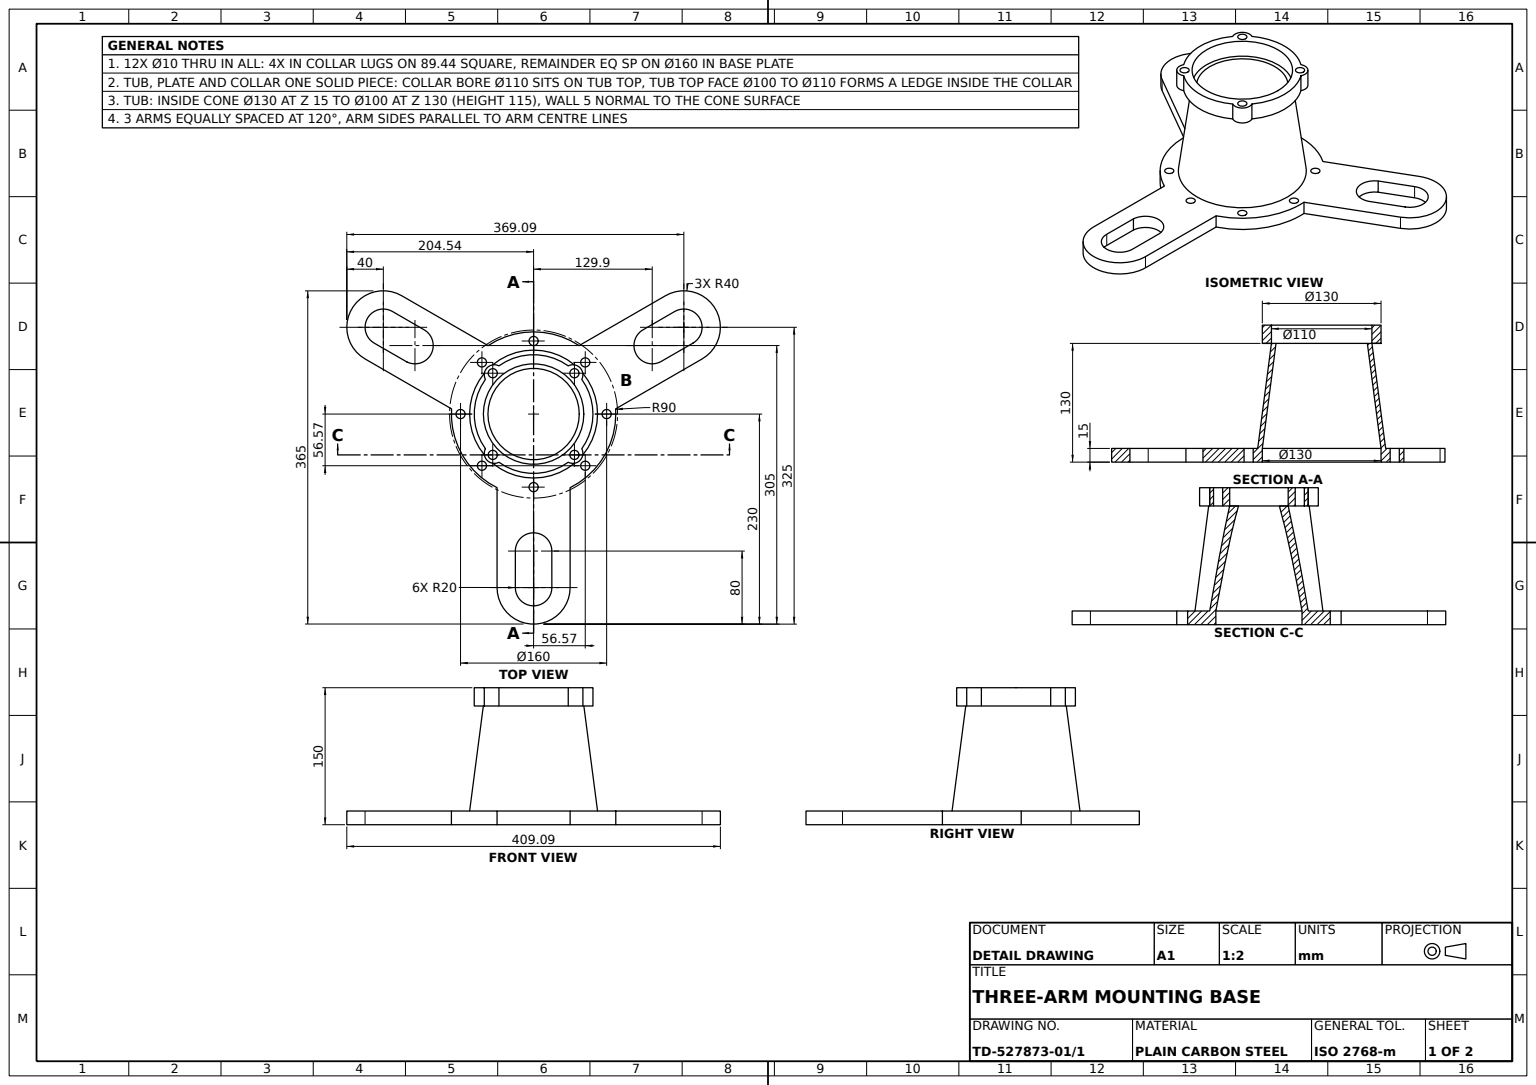
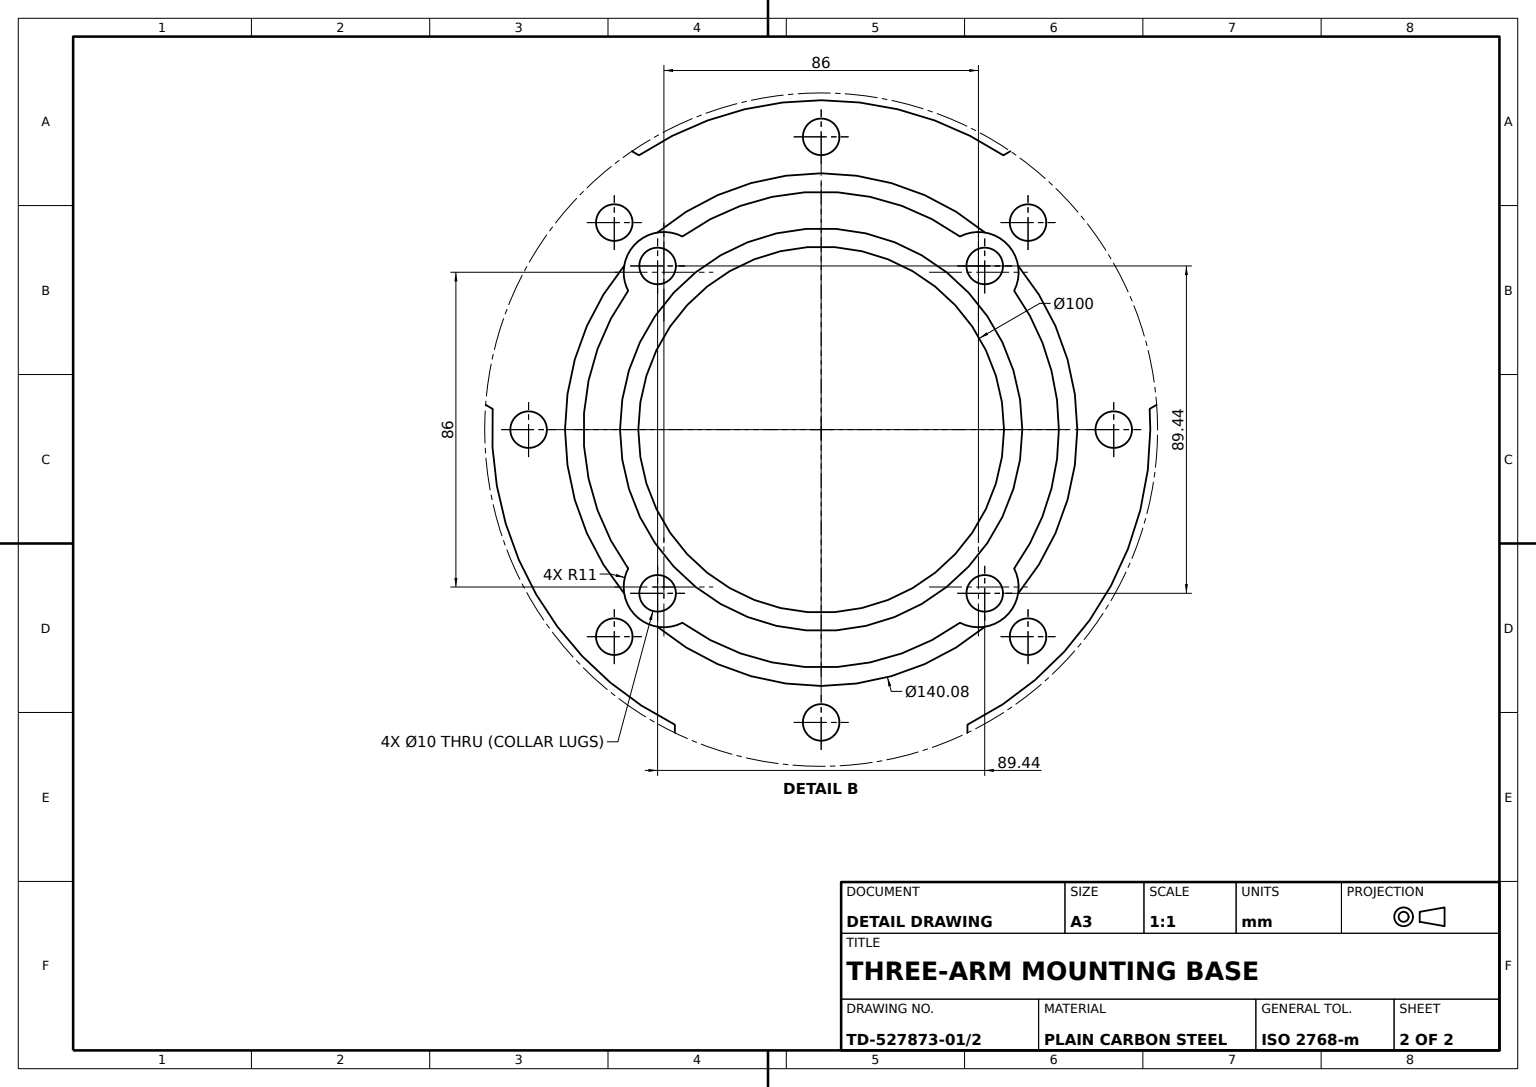
solid
v1 (-129.641016,15,-144.544827)
v2 (-74.952305,15,-49.8212)
e1 v1 v2 LINE
v3 (-129.641016,0,-144.544827)
e2 v1 v3 LINE
v4 (-74.952305,0,-49.8212)
e3 v3 v4 LINE
e4 v2 v4 LINE
face PLANE(AX(P(-34.641016,15,20),D(0.866025404,0,-0.5),D(-0.5,0,-0.866025404))) rev [-e1 e2 e3 -e4]
v5 (43,130,54)
v6 (43,150,54)
e5 v5 v6 LINE
v7 (52.771822,130,37.949109)
e6 v5 v7 CIRCLE(AX(P(43,130,43),D(0,1,0),D(-1,0,0)),11)
v8 (52.771822,150,37.949109)
e7 v8 v7 LINE
e8 v6 v8 CIRCLE(AX(P(43,150,43),D(0,1,0),D(-1,0,0)),11)
face CYL(AX(P(43,130,43),D(0,1,0),D(0,0,1)),11) [-e5 e6 -e7 -e8]
v9 (56.568542,0,-51.568542)
v10 (56.568542,15,-51.568542)
e9 v9 v10 LINE
v11 (56.568542,0,-61.568542)
e10 v11 v9 CIRCLE(AX(P(56.568542,0,-56.568542),D(0,1,0),D(0,0,1)),5)
v12 (56.568542,15,-61.568542)
e11 v11 v12 LINE
e12 v12 v10 CIRCLE(AX(P(56.568542,15,-56.568542),D(0,1,0),D(0,0,1)),5)
face CYL(AX(P(56.568542,-47,-56.568542),D(0,1,0),D(0,0,1)),5) rev [-e9 -e10 e11 e12]
v13 (0,130,-50)
v14 (0,130,50)
e13 v13 v14 CIRCLE(AX(P(0,130,0),D(0,1,0),D(0,0,1)),50)
e14 v14 v13 CIRCLE(AX(P(0,130,0),D(0,1,0),D(0,0,1)),50)
v15 (0,130,55)
v16 (0,130,-55)
e15 v15 v16 CIRCLE(AX(P(0,130,0),D(0,-1,0),D(0,0,1)),55)
e16 v16 v15 CIRCLE(AX(P(0,130,0),D(0,-1,0),D(0,0,1)),55)
face PLANE(AX(P(0,130,0),D(0,1,0),D(0,0,1))) [-e13 -e14] [-e15 -e16]
v17 (0,150,-55)
e17 v17 v16 LINE
v18 (0,150,55)
e18 v17 v18 CIRCLE(AX(P(0,150,0),D(0,1,0),D(1,0,0)),55)
e19 v18 v15 LINE
face CYL(AX(P(0,150,0),D(0,-1,0),D(0,0,-1)),55) rev [-e17 e18 e19 e15]
v19 (-44.722153,130,-49.722153)
v20 (-44.722153,150,-49.722153)
e20 v19 v20 LINE
v21 (-44.722153,130,-39.722153)
e21 v21 v19 CIRCLE(AX(P(-44.722153,130,-44.722153),D(0,1,0),D(0,0,1)),5)
v22 (-44.722153,150,-39.722153)
e22 v21 v22 LINE
e23 v22 v20 CIRCLE(AX(P(-44.722153,150,-44.722153),D(0,1,0),D(0,0,1)),5)
face CYL(AX(P(-44.722153,115,-44.722153),D(0,1,0),D(0,0,1)),5) rev [-e20 -e21 e22 e23]
v23 (148.666667,15,-19.955506)
v24 (148.666667,0,-19.955506)
e24 v23 v24 LINE
v25 (189.956941,0,-19.999954)
e25 v24 v25 LINE
v26 (189.956941,15,-19.999954)
e26 v26 v25 LINE
e27 v23 v26 LINE
face PLANE(AX(P(-0.021309,15,-19.795448),D(-0.001076466,0,-0.999999421),D(-0.999999421,0,0.001076466))) rev [e24 e25 -e26 -e27]
v27 (190,0,-20)
e28 v27 v25 CIRCLE(AX(P(190,0,0),D(0,1,0),D(0,0,1)),20)
v28 (190,15,-20)
e29 v28 v27 LINE
e30 v28 v26 CIRCLE(AX(P(190,15,0),D(0,1,0),D(0,0,1)),20)
face CYL(AX(P(190,15,0),D(0,-1,0),D(0,0,-1)),20) rev [-e28 -e29 e30 e26]
v29 (190,15,-40)
v30 (190,0,-40)
e31 v29 v30 LINE
v31 (190,15,40)
e32 v31 v29 CIRCLE(AX(P(190,15,0),D(0,1,0),D(0,0,1)),40)
v32 (190,0,40)
e33 v31 v32 LINE
e34 v32 v30 CIRCLE(AX(P(190,0,0),D(0,1,0),D(0,0,1)),40)
face CYL(AX(P(190,15,0),D(0,-1,0),D(0,0,-1)),40) [-e31 -e32 e33 e34]
v33 (-57.051358,15,-138.726863)
v34 (-57.051358,0,-138.726863)
e35 v33 v34 LINE
v35 (-91.615309,0,-118.771357)
e36 v35 v34 CIRCLE(AX(P(-75,0,-129.903811),D(0,1,0),D(0,0,1)),20)
v36 (-91.615309,15,-118.771357)
e37 v36 v35 LINE
e38 v36 v33 CIRCLE(AX(P(-75,15,-129.903811),D(0,1,0),D(0,0,1)),20)
face CYL(AX(P(-75,15,-129.903811),D(0,-1,0),D(0,0,-1)),20) rev [e35 -e36 -e37 e38]
v37 (0,0,-65)
v38 (0,0,65)
e39 v37 v38 CIRCLE(AX(P(0,0,0),D(0,1,0),D(0,0,1)),65)
v39 (0,15,-65)
e40 v37 v39 LINE
v40 (0,15,65)
e41 v39 v40 CIRCLE(AX(P(0,15,0),D(0,1,0),D(0,0,1)),65)
e42 v38 v40 LINE
face CYL(AX(P(0,-5,0),D(0,1,0),D(0,0,1)),65) rev [-e39 e40 e41 -e42]
v41 (-112.298939,15,154.50756)
v42 (-112.298939,0,154.50756)
e43 v41 v42 LINE
v43 (-77.658003,15,174.507514)
e44 v41 v43 CIRCLE(AX(P(-95,15,164.544827),D(0,1,0),D(0,0,1)),20)
v44 (-77.658003,0,174.507514)
e45 v43 v44 LINE
e46 v42 v44 CIRCLE(AX(P(-95,0,164.544827),D(0,1,0),D(0,0,1)),20)
face CYL(AX(P(-95,15,164.544827),D(0,-1,0),D(0,0,-1)),20) rev [-e43 e44 e45 -e46]
v45 (52.771822,130,-37.949109)
v46 (52.771822,150,-37.949109)
e47 v45 v46 LINE
e48 v8 v46 CIRCLE(AX(P(0,150,0),D(0,1,0),D(0,0,1)),65)
e49 v7 v45 CIRCLE(AX(P(0,130,0),D(0,1,0),D(0,0,1)),65)
face CYL(AX(P(0,150,0),D(0,-1,0),D(0,0,-1)),65) [e47 -e48 e7 e49]
v47 (-77.658003,0,-174.507514)
e50 v34 v47 LINE
v48 (-77.658003,15,-174.507514)
e51 v33 v48 LINE
e52 v48 v47 LINE
face PLANE(AX(P(17.154016,15,-9.87927),D(-0.866563135,0,0.499067464),D(0.499067464,0,0.866563135))) [-e50 -e35 e51 e52]
v49 (-56.568542,0,51.568542)
v50 (-56.568542,15,51.568542)
e53 v49 v50 LINE
v51 (-56.568542,0,61.568542)
e54 v51 v49 CIRCLE(AX(P(-56.568542,0,56.568542),D(0,1,0),D(0,0,1)),5)
v52 (-56.568542,15,61.568542)
e55 v51 v52 LINE
e56 v52 v50 CIRCLE(AX(P(-56.568542,15,56.568542),D(0,1,0),D(0,0,1)),5)
face CYL(AX(P(-56.568542,-47,56.568542),D(0,1,0),D(0,0,1)),5) rev [-e53 -e54 e55 e56]
v53 (37.949109,150,-52.771822)
v54 (37.949109,130,-52.771822)
e57 v53 v54 LINE
e58 v46 v53 CIRCLE(AX(P(43,150,-43),D(0,1,0),D(0,0,1)),11)
e59 v45 v54 CIRCLE(AX(P(43,130,-43),D(0,1,0),D(0,0,1)),11)
face CYL(AX(P(43,130,-43),D(0,1,0),D(0,0,1)),11) [-e57 -e58 -e47 e59]
v55 (-112.298939,15,-154.50756)
v56 (-112.298939,0,-154.50756)
e60 v55 v56 LINE
e61 v36 v55 LINE
e62 v35 v56 LINE
face PLANE(AX(P(-17.132707,15,9.916178),D(-0.865486669,0,0.500931957),D(0.500931957,0,0.865486669))) rev [-e60 -e61 e37 e62]
v57 (37.949109,130,52.771822)
v58 (37.949109,150,52.771822)
e63 v57 v58 LINE
e64 v57 v5 CIRCLE(AX(P(43,130,43),D(0,1,0),D(-1,0,0)),11)
e65 v58 v6 CIRCLE(AX(P(43,150,43),D(0,1,0),D(-1,0,0)),11)
face CYL(AX(P(43,130,43),D(0,1,0),D(0,0,1)),11) [-e63 e64 e5 -e65]
v59 (56.568542,0,51.568542)
v60 (56.568542,0,61.568542)
e66 v59 v60 CIRCLE(AX(P(56.568542,0,56.568542),D(0,1,0),D(0,0,1)),5)
v61 (56.568542,15,51.568542)
e67 v59 v61 LINE
v62 (56.568542,15,61.568542)
e68 v61 v62 CIRCLE(AX(P(56.568542,15,56.568542),D(0,1,0),D(0,0,1)),5)
e69 v60 v62 LINE
face CYL(AX(P(56.568542,-47,56.568542),D(0,1,0),D(0,0,1)),5) rev [-e66 e67 e68 -e69]
v63 (0,0,-75)
v64 (0,15,-75)
e70 v63 v64 LINE
v65 (0,15,-85)
e71 v64 v65 CIRCLE(AX(P(0,15,-80),D(0,1,0),D(0,0,1)),5)
v66 (0,0,-85)
e72 v66 v65 LINE
e73 v63 v66 CIRCLE(AX(P(0,0,-80),D(0,1,0),D(0,0,1)),5)
face CYL(AX(P(0,-47,-80),D(0,1,0),D(0,0,1)),5) rev [e70 e71 -e72 -e73]
v67 (44.722153,130,-49.722153)
v68 (44.722153,130,-39.722153)
e74 v67 v68 CIRCLE(AX(P(44.722153,130,-44.722153),D(0,1,0),D(0,0,1)),5)
v69 (44.722153,150,-49.722153)
e75 v67 v69 LINE
v70 (44.722153,150,-39.722153)
e76 v69 v70 CIRCLE(AX(P(44.722153,150,-44.722153),D(0,1,0),D(0,0,1)),5)
e77 v68 v70 LINE
face CYL(AX(P(44.722153,115,-44.722153),D(0,1,0),D(0,0,1)),5) rev [-e74 e75 e76 -e77]
v71 (0,130,55.042354)
v72 (0,130,-55.042354)
e78 v71 v72 CIRCLE(AX(P(0,130,0),D(0,1,0),D(0,0,1)),55.042354)
e79 v72 v71 CIRCLE(AX(P(0,130,0),D(0,1,0),D(0,0,1)),55.042354)
e80 v68 v67 CIRCLE(AX(P(44.722153,130,-44.722153),D(0,1,0),D(0,0,1)),5)
v73 (44.722153,130,49.722153)
v74 (44.722153,130,39.722153)
e81 v73 v74 CIRCLE(AX(P(44.722153,130,44.722153),D(0,1,0),D(0,0,1)),5)
e82 v74 v73 CIRCLE(AX(P(44.722153,130,44.722153),D(0,1,0),D(0,0,1)),5)
v75 (-37.949109,130,52.771822)
e83 v75 v57 CIRCLE(AX(P(0,130,0),D(0,1,0),D(0,0,1)),65)
v76 (-43,130,54)
e84 v76 v75 CIRCLE(AX(P(-43,130,43),D(0,1,0),D(0,0,-1)),11)
v77 (-52.771822,130,37.949109)
e85 v77 v76 CIRCLE(AX(P(-43,130,43),D(0,1,0),D(0,0,-1)),11)
v78 (-52.771822,130,-37.949109)
e86 v78 v77 CIRCLE(AX(P(0,130,0),D(0,1,0),D(0,0,1)),65)
v79 (-37.949109,130,-52.771822)
e87 v79 v78 CIRCLE(AX(P(-43,130,-43),D(0,1,0),D(1,0,0)),11)
v80 (0,130,-65)
e88 v80 v79 CIRCLE(AX(P(0,130,0),D(0,1,0),D(0,0,1)),65)
e89 v54 v80 CIRCLE(AX(P(0,130,0),D(0,1,0),D(0,0,1)),65)
e90 v19 v21 CIRCLE(AX(P(-44.722153,130,-44.722153),D(0,1,0),D(0,0,1)),5)
v81 (-44.722153,130,39.722153)
v82 (-44.722153,130,49.722153)
e91 v81 v82 CIRCLE(AX(P(-44.722153,130,44.722153),D(0,1,0),D(0,0,1)),5)
e92 v82 v81 CIRCLE(AX(P(-44.722153,130,44.722153),D(0,1,0),D(0,0,1)),5)
face PLANE(AX(P(0,130,0),D(0,1,0),D(0,0,1))) rev [e78 e79] [e80 e74] [e81 e82] [-e59 -e49 -e6 -e64 -e83 -e84 -e85 -e86 -e87 -e88 -e89] [e90 e21] [e91 e92]
v83 (-43,150,54)
e93 v76 v83 LINE
v84 (-37.949109,150,52.771822)
e94 v84 v75 LINE
e95 v83 v84 CIRCLE(AX(P(-43,150,43),D(0,1,0),D(0,0,-1)),11)
face CYL(AX(P(-43,130,43),D(0,1,0),D(0,0,1)),11) [-e93 e84 -e94 -e95]
v85 (-57.051358,0,138.726863)
v86 (-75,0,109.903811)
e96 v85 v86 CIRCLE(AX(P(-75,0,129.903811),D(0,1,0),D(0,0,1)),20)
v87 (-57.051358,15,138.726863)
e97 v87 v85 LINE
v88 (-75,15,109.903811)
e98 v87 v88 CIRCLE(AX(P(-75,15,129.903811),D(0,1,0),D(0,0,1)),20)
e99 v88 v86 LINE
face CYL(AX(P(-75,15,129.903811),D(0,-1,0),D(0,0,-1)),20) rev [-e96 -e97 e98 e99]
v89 (0,15,70.042354)
e100 v71 v89 LINE
v90 (0,15,-70.042354)
e101 v89 v90 CIRCLE(AX(P(0,15,0),D(0,1,0),D(0,0,1)),70.042354)
e102 v72 v90 LINE
face CONE(AX(P(0,130.646696,0),D(0,-1,0),D(0,0,-1)),54.958002056,0.129702537) [-e78 e100 e101 -e102]
v91 (-44.722153,150,39.722153)
e103 v81 v91 LINE
v92 (-44.722153,150,49.722153)
e104 v91 v92 CIRCLE(AX(P(-44.722153,150,44.722153),D(0,1,0),D(0,0,1)),5)
e105 v82 v92 LINE
face CYL(AX(P(-44.722153,115,44.722153),D(0,1,0),D(0,0,1)),5) rev [-e91 e103 e104 -e105]
e106 v13 v39 LINE
e107 v40 v39 CIRCLE(AX(P(0,15,0),D(0,1,0),D(0,0,1)),65)
e108 v14 v40 LINE
face CONE(AX(P(0,130,0),D(0,-1,0),D(0,0,-1)),50,0.129702537) rev [e106 -e107 -e108 e14]
v93 (-74.952305,15,49.8212)
v94 (-74.952305,0,49.8212)
e109 v93 v94 LINE
v95 (-129.641016,0,144.544827)
e110 v95 v94 LINE
v96 (-129.641016,15,144.544827)
e111 v96 v95 LINE
e112 v96 v93 LINE
face PLANE(AX(P(-34.641016,15,-20),D(-0.866025404,0,-0.5),D(-0.5,0,0.866025404))) [e109 -e110 -e111 e112]
v97 (80,15,-5)
v98 (80,15,5)
e113 v97 v98 CIRCLE(AX(P(80,15,0),D(0,1,0),D(0,0,1)),5)
v99 (80,0,5)
e114 v99 v98 LINE
v100 (80,0,-5)
e115 v100 v99 CIRCLE(AX(P(80,0,0),D(0,1,0),D(0,0,1)),5)
e116 v100 v97 LINE
face CYL(AX(P(80,-47,0),D(0,1,0),D(0,0,1)),5) rev [e113 -e114 -e115 e116]
v101 (-95,0,-184.544827)
e117 v101 v56 CIRCLE(AX(P(-95,0,-164.544827),D(0,1,0),D(0,0,1)),20)
v102 (-95,15,-184.544827)
e118 v102 v101 LINE
e119 v102 v55 CIRCLE(AX(P(-95,15,-164.544827),D(0,1,0),D(0,0,1)),20)
face CYL(AX(P(-95,15,-164.544827),D(0,-1,0),D(0,0,-1)),20) rev [e60 -e117 -e118 e119]
e120 v84 v58 CIRCLE(AX(P(0,150,0),D(0,1,0),D(0,0,1)),65)
face CYL(AX(P(0,150,0),D(0,-1,0),D(0,0,-1)),65) [e94 e83 e63 -e120]
e121 v18 v17 CIRCLE(AX(P(0,150,0),D(0,1,0),D(1,0,0)),55)
face CYL(AX(P(0,150,0),D(0,-1,0),D(0,0,-1)),55) rev [-e19 e121 e17 e16]
e122 v98 v97 CIRCLE(AX(P(80,15,0),D(0,1,0),D(0,0,1)),5)
v103 (0,15,85)
v104 (0,15,75)
e123 v103 v104 CIRCLE(AX(P(0,15,80),D(0,1,0),D(0,0,1)),5)
e124 v104 v103 CIRCLE(AX(P(0,15,80),D(0,1,0),D(0,0,1)),5)
e125 v48 v102 CIRCLE(AX(P(-95,15,-164.544827),D(0,1,0),D(0,0,1)),20)
v105 (-56.568542,15,-51.568542)
v106 (-56.568542,15,-61.568542)
e126 v105 v106 CIRCLE(AX(P(-56.568542,15,-56.568542),D(0,1,0),D(0,0,1)),5)
e127 v106 v105 CIRCLE(AX(P(-56.568542,15,-56.568542),D(0,1,0),D(0,0,1)),5)
e128 v50 v52 CIRCLE(AX(P(-56.568542,15,56.568542),D(0,1,0),D(0,0,1)),5)
e129 v65 v64 CIRCLE(AX(P(0,15,-80),D(0,1,0),D(0,0,1)),5)
e130 v90 v89 CIRCLE(AX(P(0,15,0),D(0,1,0),D(0,0,1)),70.042354)
v107 (190,15,20)
e131 v107 v28 CIRCLE(AX(P(190,15,0),D(0,1,0),D(0,0,1)),20)
v108 (189.956941,15,19.999954)
e132 v108 v107 CIRCLE(AX(P(190,15,0),D(0,1,0),D(0,0,1)),20)
v109 (148.666667,15,19.955506)
e133 v109 v108 LINE
e134 v23 v109 CIRCLE(AX(P(150,15,0),D(0,1,0),D(0,0,1)),20)
e135 v2 v93 CIRCLE(AX(P(0,15,0),D(0,1,0),D(0,0,1)),90)
v110 (-60.358984,15,184.544827)
e136 v96 v110 CIRCLE(AX(P(-95,15,164.544827),D(0,1,0),D(0,0,1)),40)
v111 (-5.670273,15,89.8212)
e137 v110 v111 LINE
v112 (80.622577,15,40)
e138 v111 v112 CIRCLE(AX(P(0,15,0),D(0,1,0),D(0,0,1)),90)
e139 v31 v112 LINE
v113 (80.622577,15,-40)
e140 v29 v113 LINE
v114 (0,15,-90)
e141 v113 v114 CIRCLE(AX(P(0,15,0),D(0,1,0),D(0,0,1)),90)
v115 (-5.670273,15,-89.8212)
e142 v114 v115 CIRCLE(AX(P(0,15,0),D(0,1,0),D(0,0,1)),90)
v116 (-60.358984,15,-184.544827)
e143 v116 v115 LINE
v117 (-95,15,-204.544827)
e144 v116 v117 CIRCLE(AX(P(-95,15,-164.544827),D(0,1,0),D(0,0,1)),40)
e145 v117 v1 CIRCLE(AX(P(-95,15,-164.544827),D(0,1,0),D(0,0,1)),40)
e146 v10 v12 CIRCLE(AX(P(56.568542,15,-56.568542),D(0,1,0),D(0,0,1)),5)
v118 (-80,15,-5)
v119 (-80,15,5)
e147 v118 v119 CIRCLE(AX(P(-80,15,0),D(0,1,0),D(0,0,1)),5)
e148 v119 v118 CIRCLE(AX(P(-80,15,0),D(0,1,0),D(0,0,1)),5)
v120 (-91.615309,15,118.771357)
e149 v88 v120 CIRCLE(AX(P(-75,15,129.903811),D(0,1,0),D(0,0,1)),20)
e150 v87 v43 LINE
e151 v120 v41 LINE
e152 v62 v61 CIRCLE(AX(P(56.568542,15,56.568542),D(0,1,0),D(0,0,1)),5)
face PLANE(AX(P(0,15,0),D(0,1,0),D(0,0,1))) [-e113 -e122] [-e123 -e124] [-e125 -e51 -e38 e61 -e119] [-e126 -e127] [-e56 -e128] [-e71 -e129] [-e130 -e101] [-e131 -e132 -e133 -e134 e27 -e30] [e135 -e112 e136 e137 e138 -e139 e32 e140 e141 e142 -e143 e144 e145 e1] [-e146 -e12] [-e147 -e148] [-e149 -e98 e150 -e44 -e151] [-e152 -e68]
v121 (-91.615309,0,118.771357)
e153 v86 v121 CIRCLE(AX(P(-75,0,129.903811),D(0,1,0),D(0,0,1)),20)
e154 v121 v42 LINE
e155 v85 v44 LINE
v122 (-60.358984,0,-184.544827)
v123 (-5.670273,0,-89.8212)
e156 v122 v123 LINE
v124 (0,0,-90)
e157 v124 v123 CIRCLE(AX(P(0,0,0),D(0,1,0),D(0,0,1)),90)
v125 (80.622577,0,-40)
e158 v125 v124 CIRCLE(AX(P(0,0,0),D(0,1,0),D(0,0,1)),90)
e159 v30 v125 LINE
v126 (80.622577,0,40)
e160 v32 v126 LINE
v127 (-5.670273,0,89.8212)
e161 v127 v126 CIRCLE(AX(P(0,0,0),D(0,1,0),D(0,0,1)),90)
v128 (-60.358984,0,184.544827)
e162 v128 v127 LINE
e163 v95 v128 CIRCLE(AX(P(-95,0,164.544827),D(0,1,0),D(0,0,1)),40)
e164 v4 v94 CIRCLE(AX(P(0,0,0),D(0,1,0),D(0,0,1)),90)
v129 (-95,0,-204.544827)
e165 v129 v3 CIRCLE(AX(P(-95,0,-164.544827),D(0,1,0),D(0,0,1)),40)
e166 v122 v129 CIRCLE(AX(P(-95,0,-164.544827),D(0,1,0),D(0,0,1)),40)
v130 (0,0,75)
v131 (0,0,85)
e167 v130 v131 CIRCLE(AX(P(0,0,80),D(0,1,0),D(0,0,1)),5)
e168 v131 v130 CIRCLE(AX(P(0,0,80),D(0,1,0),D(0,0,1)),5)
v132 (-56.568542,0,-61.568542)
v133 (-56.568542,0,-51.568542)
e169 v132 v133 CIRCLE(AX(P(-56.568542,0,-56.568542),D(0,1,0),D(0,0,1)),5)
e170 v133 v132 CIRCLE(AX(P(-56.568542,0,-56.568542),D(0,1,0),D(0,0,1)),5)
e171 v66 v63 CIRCLE(AX(P(0,0,-80),D(0,1,0),D(0,0,1)),5)
e172 v38 v37 CIRCLE(AX(P(0,0,0),D(0,1,0),D(0,0,1)),65)
e173 v47 v101 CIRCLE(AX(P(-95,0,-164.544827),D(0,1,0),D(0,0,1)),20)
e174 v60 v59 CIRCLE(AX(P(56.568542,0,56.568542),D(0,1,0),D(0,0,1)),5)
e175 v49 v51 CIRCLE(AX(P(-56.568542,0,56.568542),D(0,1,0),D(0,0,1)),5)
v134 (148.666667,0,19.955506)
e176 v24 v134 CIRCLE(AX(P(150,0,0),D(0,1,0),D(0,0,1)),20)
v135 (189.956941,0,19.999954)
e177 v134 v135 LINE
v136 (190,0,20)
e178 v135 v136 CIRCLE(AX(P(190,0,0),D(0,1,0),D(0,0,1)),20)
e179 v136 v27 CIRCLE(AX(P(190,0,0),D(0,1,0),D(0,0,1)),20)
e180 v9 v11 CIRCLE(AX(P(56.568542,0,-56.568542),D(0,1,0),D(0,0,1)),5)
v137 (-80,0,5)
v138 (-80,0,-5)
e181 v137 v138 CIRCLE(AX(P(-80,0,0),D(0,1,0),D(0,0,1)),5)
e182 v138 v137 CIRCLE(AX(P(-80,0,0),D(0,1,0),D(0,0,1)),5)
e183 v99 v100 CIRCLE(AX(P(80,0,0),D(0,1,0),D(0,0,1)),5)
face PLANE(AX(P(0,0,0),D(0,1,0),D(0,0,1))) rev [e96 e153 e154 e46 -e155] [e156 -e157 -e158 -e159 -e34 e160 -e161 -e162 -e163 e110 -e164 -e3 -e165 -e166] [e167 e168] [e169 e170] [e73 e171] [e172 e39] [e36 e50 e173 e117 -e62] [e66 e174] [e54 e175] [e28 -e25 e176 e177 e178 e179] [e10 e180] [e181 e182] [e115 e183]
e184 v115 v123 LINE
e185 v116 v122 LINE
face PLANE(AX(P(34.641016,15,-20),D(0.866025404,0,-0.5),D(-0.5,0,-0.866025404))) [e184 -e156 -e185 e143]
v139 (-37.949109,150,-52.771822)
e186 v79 v139 LINE
v140 (-52.771822,150,-37.949109)
e187 v140 v78 LINE
e188 v139 v140 CIRCLE(AX(P(-43,150,-43),D(0,1,0),D(1,0,0)),11)
face CYL(AX(P(-43,130,-43),D(0,1,0),D(0,0,1)),11) [-e186 e87 -e187 -e188]
face CYL(AX(P(-95,15,-164.544827),D(0,-1,0),D(0,0,-1)),20) rev [e118 -e173 -e52 e125]
e189 v70 v69 CIRCLE(AX(P(44.722153,150,-44.722153),D(0,1,0),D(0,0,1)),5)
face CYL(AX(P(44.722153,115,-44.722153),D(0,1,0),D(0,0,1)),5) rev [e189 -e75 -e80 e77]
v141 (-52.771822,150,37.949109)
e190 v141 v83 CIRCLE(AX(P(-43,150,43),D(0,1,0),D(0,0,-1)),11)
e191 v77 v141 LINE
face CYL(AX(P(-43,130,43),D(0,1,0),D(0,0,1)),11) [e85 e93 -e190 -e191]
e192 v133 v105 LINE
e193 v132 v106 LINE
face CYL(AX(P(-56.568542,-47,-56.568542),D(0,1,0),D(0,0,1)),5) rev [-e192 -e169 e193 e127]
e194 v112 v126 LINE
e195 v111 v127 LINE
face CYL(AX(P(0,15,0),D(0,-1,0),D(0,0,-1)),90) [e161 -e194 -e138 e195]
face CYL(AX(P(80,-47,0),D(0,1,0),D(0,0,1)),5) rev [-e116 -e183 e114 e122]
e196 v113 v125 LINE
face PLANE(AX(P(0,15,-40),D(0,0,1),D(1,0,0))) rev [e31 e159 -e196 -e140]
v142 (44.722153,150,39.722153)
e197 v74 v142 LINE
v143 (44.722153,150,49.722153)
e198 v142 v143 CIRCLE(AX(P(44.722153,150,44.722153),D(0,1,0),D(0,0,1)),5)
e199 v73 v143 LINE
face CYL(AX(P(44.722153,115,44.722153),D(0,1,0),D(0,0,1)),5) rev [e197 e198 -e199 -e82]
v144 (0,150,-65)
e200 v144 v80 LINE
e201 v53 v144 CIRCLE(AX(P(0,150,0),D(0,1,0),D(0,0,1)),65)
face CYL(AX(P(0,150,0),D(0,-1,0),D(0,0,-1)),65) [-e200 -e201 e57 e89]
e202 v20 v22 CIRCLE(AX(P(-44.722153,150,-44.722153),D(0,1,0),D(0,0,1)),5)
face CYL(AX(P(-44.722153,115,-44.722153),D(0,1,0),D(0,0,1)),5) rev [-e90 e20 e202 -e22]
e203 v114 v124 LINE
face CYL(AX(P(0,15,0),D(0,-1,0),D(0,0,-1)),90) [-e142 e203 e157 -e184]
e204 v117 v129 LINE
face CYL(AX(P(-95,15,-164.544827),D(0,-1,0),D(0,0,-1)),40) [-e2 -e145 e204 e165]
e205 v143 v142 CIRCLE(AX(P(44.722153,150,44.722153),D(0,1,0),D(0,0,1)),5)
face CYL(AX(P(44.722153,115,44.722153),D(0,1,0),D(0,0,1)),5) rev [-e81 e199 e205 -e197]
face CYL(AX(P(0,15,0),D(0,-1,0),D(0,0,-1)),90) [-e135 e4 e164 -e109]
e206 v107 v136 LINE
face CYL(AX(P(190,15,0),D(0,-1,0),D(0,0,-1)),20) rev [e131 e29 -e179 -e206]
face PLANE(AX(P(17.154016,15,9.87927),D(0.866563135,0,0.499067464),D(0.499067464,0,-0.866563135))) rev [-e150 e97 e155 -e45]
e207 v92 v91 CIRCLE(AX(P(-44.722153,150,44.722153),D(0,1,0),D(0,0,1)),5)
face CYL(AX(P(-44.722153,115,44.722153),D(0,1,0),D(0,0,1)),5) rev [e105 e207 -e103 -e92]
face CYL(AX(P(0,-5,0),D(0,1,0),D(0,0,1)),65) rev [e107 -e40 -e172 e42]
e208 v120 v121 LINE
face PLANE(AX(P(-17.132707,15,-9.916178),D(0.865486669,0,0.500931957),D(0.500931957,0,-0.865486669))) [e43 -e154 -e208 e151]
face CYL(AX(P(-56.568542,-47,56.568542),D(0,1,0),D(0,0,1)),5) rev [e53 e128 -e55 -e175]
face CYL(AX(P(56.568542,-47,56.568542),D(0,1,0),D(0,0,1)),5) rev [e69 e152 -e67 -e174]
e209 v144 v139 CIRCLE(AX(P(0,150,0),D(0,1,0),D(0,0,1)),65)
face CYL(AX(P(0,150,0),D(0,-1,0),D(0,0,-1)),65) [e186 -e209 e200 e88]
e210 v131 v103 LINE
e211 v130 v104 LINE
face CYL(AX(P(0,-47,80),D(0,1,0),D(0,0,1)),5) rev [e124 -e210 -e167 e211]
face CONE(AX(P(0,130,0),D(0,-1,0),D(0,0,-1)),50,0.129702537) rev [e108 -e41 -e106 e13]
face CYL(AX(P(56.568542,-47,-56.568542),D(0,1,0),D(0,0,1)),5) rev [-e180 e9 e146 -e11]
e212 v110 v128 LINE
face PLANE(AX(P(34.641016,15,20),D(-0.866025404,0,-0.5),D(-0.5,0,0.866025404))) rev [e162 -e195 -e137 e212]
e213 v140 v141 CIRCLE(AX(P(0,150,0),D(0,1,0),D(0,0,1)),65)
face CYL(AX(P(0,150,0),D(0,-1,0),D(0,0,-1)),65) [e187 e86 e191 -e213]
face CYL(AX(P(-95,15,164.544827),D(0,-1,0),D(0,0,-1)),40) [e163 -e212 -e136 e111]
face CYL(AX(P(0,15,0),D(0,-1,0),D(0,0,-1)),90) [e158 -e203 -e141 e196]
face PLANE(AX(P(0,15,40),D(0,0,1),D(1,0,0))) [e194 -e160 -e33 e139]
face CYL(AX(P(-56.568542,-47,-56.568542),D(0,1,0),D(0,0,1)),5) rev [-e193 -e170 e192 e126]
face PLANE(AX(P(0,150,0),D(0,1,0),D(0,0,1))) [e65 e8 e48 e58 e201 e209 e188 e213 e190 e95 e120] [-e202 -e23] [-e76 -e189] [-e205 -e198] [-e18 -e121] [-e207 -e104]
face CONE(AX(P(0,130.646696,0),D(0,-1,0),D(0,0,-1)),54.958002056,0.129702537) [-e79 e102 e130 -e100]
e214 v108 v135 LINE
face CYL(AX(P(190,15,0),D(0,-1,0),D(0,0,-1)),20) rev [-e214 e132 e206 -e178]
e215 v138 v118 LINE
e216 v137 v119 LINE
face CYL(AX(P(-80,-47,0),D(0,1,0),D(0,0,1)),5) rev [-e215 -e181 e216 e148]
face CYL(AX(P(-95,15,-164.544827),D(0,-1,0),D(0,0,-1)),40) [-e204 -e144 e185 e166]
face CYL(AX(P(-80,-47,0),D(0,1,0),D(0,0,1)),5) rev [-e182 e215 e147 -e216]
face CYL(AX(P(0,-47,-80),D(0,1,0),D(0,0,1)),5) rev [-e171 e72 e129 -e70]
e217 v109 v134 LINE
face CYL(AX(P(150,15,0),D(0,-1,0),D(0,0,-1)),20) rev [e134 e217 -e176 -e24]
face PLANE(AX(P(-0.021309,15,19.795448),D(0.001076466,0,-0.999999421),D(-0.999999421,0,-0.001076466))) [e214 -e177 -e217 e133]
face CYL(AX(P(-75,15,129.903811),D(0,-1,0),D(0,0,-1)),20) rev [e208 -e153 -e99 e149]
face CYL(AX(P(0,-47,80),D(0,1,0),D(0,0,1)),5) rev [-e211 -e168 e210 e123]
